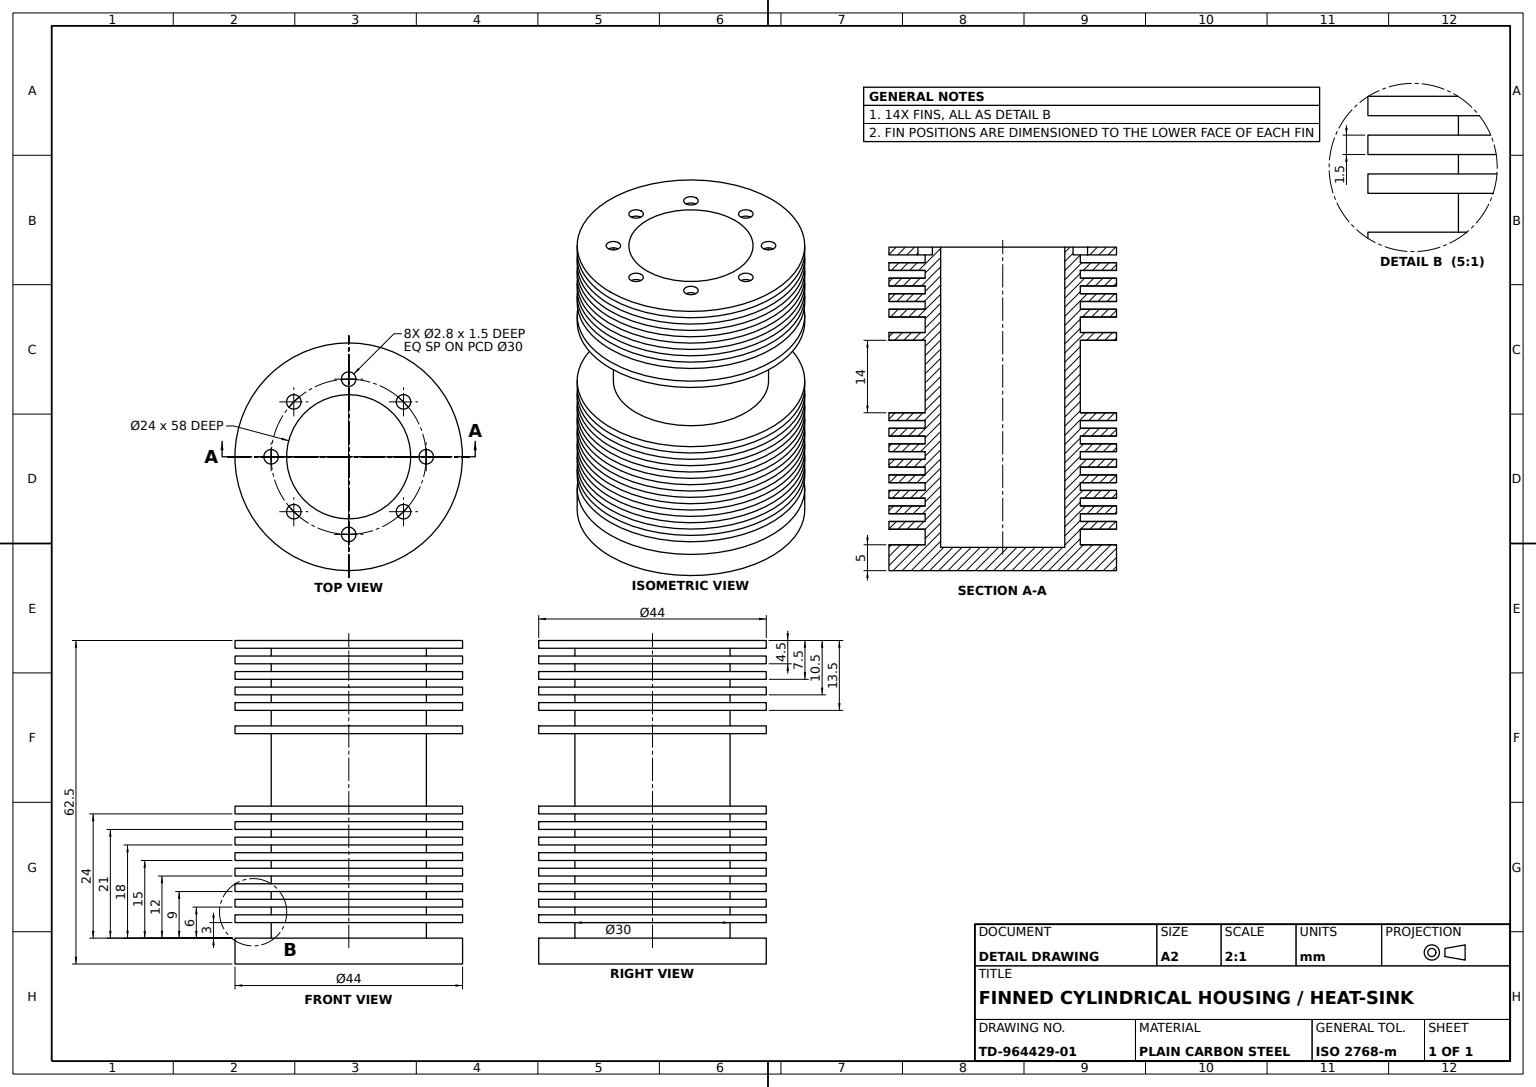
solid
v1 (0,61,13.6)
v2 (0,62.5,13.6)
e1 v1 v2 LINE
v3 (0,62.5,16.4)
e2 v2 v3 CIRCLE(AX(P(0,62.5,15),D(0,1,0),D(0,0,1)),1.4)
v4 (0,61,16.4)
e3 v4 v3 LINE
v5 (-1.398475,61,14.934667)
e4 v5 v4 CIRCLE(AX(P(0,61,15),D(0,1,0),D(0,0,1)),1.4)
e5 v1 v5 CIRCLE(AX(P(0,61,15),D(0,1,0),D(0,0,1)),1.4)
face CYL(AX(P(0,61,15),D(0,1,0),D(0,0,1)),1.4) rev [e1 e2 -e3 -e4 -e5]
v6 (0,15.5,22)
v7 (0,14,22)
e6 v6 v7 LINE
v8 (0,15.5,-22)
e7 v8 v6 CIRCLE(AX(P(0,15.5,0),D(0,1,0),D(0,0,1)),22)
v9 (0,14,-22)
e8 v8 v9 LINE
e9 v9 v7 CIRCLE(AX(P(0,14,0),D(0,1,0),D(0,0,1)),22)
face CYL(AX(P(0,15.5,0),D(0,-1,0),D(0,0,-1)),22) [-e6 -e7 e8 e9]
v10 (0,52,-22)
v11 (0,52,22)
e10 v10 v11 CIRCLE(AX(P(0,52,0),D(0,1,0),D(0,0,1)),22)
v12 (0,53.5,22)
e11 v12 v11 LINE
v13 (0,53.5,-22)
e12 v13 v12 CIRCLE(AX(P(0,53.5,0),D(0,1,0),D(0,0,1)),22)
e13 v13 v10 LINE
face CYL(AX(P(0,53.5,0),D(0,-1,0),D(0,0,-1)),22) [e10 -e11 -e12 e13]
v14 (0,4.5,-12)
v15 (0,4.5,12)
e14 v14 v15 CIRCLE(AX(P(0,4.5,0),D(0,1,0),D(0,0,1)),12)
e15 v15 v14 CIRCLE(AX(P(0,4.5,0),D(0,1,0),D(0,0,1)),12)
face PLANE(AX(P(0,4.5,0),D(0,1,0),D(0,0,1))) [e14 e15]
v16 (0,21.5,15)
v17 (0,21.5,-15)
e16 v16 v17 CIRCLE(AX(P(0,21.5,0),D(0,1,0),D(0,0,1)),15)
v18 (0,23,-15)
e17 v17 v18 LINE
v19 (0,23,15)
e18 v19 v18 CIRCLE(AX(P(0,23,0),D(0,1,0),D(0,0,1)),15)
e19 v16 v19 LINE
face CYL(AX(P(0,4.5,0),D(0,1,0),D(0,0,1)),15) [e16 e17 -e18 -e19]
v20 (-14.934667,61,-1.398475)
v21 (-14.934667,61,1.398475)
e20 v20 v21 CIRCLE(AX(P(0,61,0),D(0,1,0),D(0,0,1)),15)
e21 v21 v20 CIRCLE(AX(P(-15,61,0),D(0,1,0),D(0,0,1)),1.4)
face PLANE(AX(P(-15,61,0),D(0,1,0),D(0,0,1))) [e20 e21]
v22 (10.606602,61,-9.206602)
v23 (11.549275,61,-9.571533)
e22 v22 v23 CIRCLE(AX(P(10.606602,61,-10.606602),D(0,1,0),D(0,0,1)),1.4)
v24 (9.571533,61,-11.549275)
e23 v23 v24 CIRCLE(AX(P(0,61,0),D(0,1,0),D(0,0,1)),15)
e24 v24 v22 CIRCLE(AX(P(10.606602,61,-10.606602),D(0,1,0),D(0,0,1)),1.4)
face PLANE(AX(P(10.606602,61,-10.606602),D(0,1,0),D(0,0,1))) [e22 e23 e24]
v25 (-10.606602,61,9.206602)
v26 (-11.549275,61,9.571533)
e25 v25 v26 CIRCLE(AX(P(-10.606602,61,10.606602),D(0,1,0),D(0,0,1)),1.4)
v27 (-10.606602,62.5,9.206602)
e26 v25 v27 LINE
v28 (-10.606602,62.5,12.006602)
e27 v27 v28 CIRCLE(AX(P(-10.606602,62.5,10.606602),D(0,1,0),D(0,0,1)),1.4)
v29 (-10.606602,61,12.006602)
e28 v29 v28 LINE
e29 v26 v29 CIRCLE(AX(P(-10.606602,61,10.606602),D(0,1,0),D(0,0,1)),1.4)
face CYL(AX(P(-10.606602,61,10.606602),D(0,1,0),D(0,0,1)),1.4) rev [-e25 e26 e27 -e28 -e29]
v30 (-9.571533,61,-11.549275)
v31 (-11.549275,61,-9.571533)
e30 v30 v31 CIRCLE(AX(P(0,61,0),D(0,1,0),D(0,0,1)),15)
v32 (-10.606602,61,-9.206602)
e31 v31 v32 CIRCLE(AX(P(-10.606602,61,-10.606602),D(0,1,0),D(0,0,1)),1.4)
e32 v32 v30 CIRCLE(AX(P(-10.606602,61,-10.606602),D(0,1,0),D(0,0,1)),1.4)
face PLANE(AX(P(-10.606602,61,-10.606602),D(0,1,0),D(0,0,1))) [e30 e31 e32]
v33 (0,50.5,-15)
v34 (0,52,-15)
e33 v33 v34 LINE
v35 (0,52,15)
e34 v35 v34 CIRCLE(AX(P(0,52,0),D(0,1,0),D(0,0,1)),15)
v36 (0,50.5,15)
e35 v36 v35 LINE
e36 v36 v33 CIRCLE(AX(P(0,50.5,0),D(0,1,0),D(0,0,1)),15)
face CYL(AX(P(0,4.5,0),D(0,1,0),D(0,0,1)),15) [e33 -e34 -e35 e36]
e37 v12 v13 CIRCLE(AX(P(0,53.5,0),D(0,1,0),D(0,0,1)),22)
e38 v11 v10 CIRCLE(AX(P(0,52,0),D(0,1,0),D(0,0,1)),22)
face CYL(AX(P(0,53.5,0),D(0,-1,0),D(0,0,-1)),22) [-e13 -e37 e11 e38]
v37 (-15,61,-1.4)
e39 v20 v37 CIRCLE(AX(P(-15,61,0),D(0,1,0),D(0,0,1)),1.4)
v38 (-15,61,1.4)
e40 v37 v38 CIRCLE(AX(P(-15,61,0),D(0,1,0),D(0,0,1)),1.4)
e41 v38 v21 CIRCLE(AX(P(-15,61,0),D(0,1,0),D(0,0,1)),1.4)
e42 v21 v26 CIRCLE(AX(P(0,61,0),D(0,1,0),D(0,0,1)),15)
v39 (-9.571533,61,11.549275)
e43 v29 v39 CIRCLE(AX(P(-10.606602,61,10.606602),D(0,1,0),D(0,0,1)),1.4)
e44 v39 v5 CIRCLE(AX(P(0,61,0),D(0,1,0),D(0,0,1)),15)
v40 (1.398475,61,14.934667)
e45 v4 v40 CIRCLE(AX(P(0,61,15),D(0,1,0),D(0,0,1)),1.4)
v41 (9.571533,61,11.549275)
e46 v40 v41 CIRCLE(AX(P(0,61,0),D(0,1,0),D(0,0,1)),15)
v42 (10.606602,61,12.006602)
e47 v41 v42 CIRCLE(AX(P(10.606602,61,10.606602),D(0,1,0),D(0,0,1)),1.4)
v43 (11.549275,61,9.571533)
e48 v42 v43 CIRCLE(AX(P(10.606602,61,10.606602),D(0,1,0),D(0,0,1)),1.4)
v44 (14.934667,61,1.398475)
e49 v43 v44 CIRCLE(AX(P(0,61,0),D(0,1,0),D(0,0,1)),15)
v45 (15,61,1.4)
e50 v44 v45 CIRCLE(AX(P(15,61,0),D(0,1,0),D(0,0,1)),1.4)
v46 (15,61,-1.4)
e51 v45 v46 CIRCLE(AX(P(15,61,0),D(0,1,0),D(0,0,1)),1.4)
v47 (14.934667,61,-1.398475)
e52 v46 v47 CIRCLE(AX(P(15,61,0),D(0,1,0),D(0,0,1)),1.4)
e53 v47 v23 CIRCLE(AX(P(0,61,0),D(0,1,0),D(0,0,1)),15)
v48 (10.606602,61,-12.006602)
e54 v23 v48 CIRCLE(AX(P(10.606602,61,-10.606602),D(0,1,0),D(0,0,1)),1.4)
e55 v48 v24 CIRCLE(AX(P(10.606602,61,-10.606602),D(0,1,0),D(0,0,1)),1.4)
v49 (1.398475,61,-14.934667)
e56 v24 v49 CIRCLE(AX(P(0,61,0),D(0,1,0),D(0,0,1)),15)
v50 (0,61,-16.4)
e57 v49 v50 CIRCLE(AX(P(0,61,-15),D(0,1,0),D(0,0,1)),1.4)
v51 (-1.398475,61,-14.934667)
e58 v50 v51 CIRCLE(AX(P(0,61,-15),D(0,1,0),D(0,0,1)),1.4)
e59 v51 v30 CIRCLE(AX(P(0,61,0),D(0,1,0),D(0,0,1)),15)
v52 (-10.606602,61,-12.006602)
e60 v30 v52 CIRCLE(AX(P(-10.606602,61,-10.606602),D(0,1,0),D(0,0,1)),1.4)
e61 v52 v31 CIRCLE(AX(P(-10.606602,61,-10.606602),D(0,1,0),D(0,0,1)),1.4)
e62 v31 v20 CIRCLE(AX(P(0,61,0),D(0,1,0),D(0,0,1)),15)
v53 (0,61,22)
v54 (0,61,-22)
e63 v53 v54 CIRCLE(AX(P(0,61,0),D(0,1,0),D(0,0,1)),22)
e64 v54 v53 CIRCLE(AX(P(0,61,0),D(0,1,0),D(0,0,1)),22)
face PLANE(AX(P(0,61,0),D(0,1,0),D(0,0,1))) rev [e39 e40 e41 e42 e29 e43 e44 e4 e45 e46 e47 e48 e49 e50 e51 e52 e53 e54 e55 e56 e57 e58 e59 e60 e61 e62] [-e63 -e64]
v55 (0,49,15)
v56 (0,49,-15)
e65 v55 v56 CIRCLE(AX(P(0,49,0),D(0,1,0),D(0,0,1)),15)
v57 (0,46,15)
e66 v57 v55 LINE
v58 (0,46,-15)
e67 v57 v58 CIRCLE(AX(P(0,46,0),D(0,1,0),D(0,0,1)),15)
e68 v58 v56 LINE
face CYL(AX(P(0,4.5,0),D(0,1,0),D(0,0,1)),15) [-e65 -e66 e67 e68]
v59 (0,21.5,22)
v60 (0,20,22)
e69 v59 v60 LINE
v61 (0,21.5,-22)
e70 v61 v59 CIRCLE(AX(P(0,21.5,0),D(0,1,0),D(0,0,1)),22)
v62 (0,20,-22)
e71 v61 v62 LINE
e72 v62 v60 CIRCLE(AX(P(0,20,0),D(0,1,0),D(0,0,1)),22)
face CYL(AX(P(0,21.5,0),D(0,-1,0),D(0,0,-1)),22) [-e69 -e70 e71 e72]
v63 (15,62.5,1.4)
e73 v45 v63 LINE
v64 (15,62.5,-1.4)
e74 v63 v64 CIRCLE(AX(P(15,62.5,0),D(0,1,0),D(0,0,1)),1.4)
e75 v46 v64 LINE
face CYL(AX(P(15,61,0),D(0,1,0),D(0,0,1)),1.4) rev [e73 e74 -e75 -e51]
v65 (0,0,22)
v66 (0,0,-22)
e76 v65 v66 CIRCLE(AX(P(0,0,0),D(0,1,0),D(0,0,1)),22)
e77 v66 v65 CIRCLE(AX(P(0,0,0),D(0,1,0),D(0,0,1)),22)
face PLANE(AX(P(0,0,0),D(0,1,0),D(0,0,1))) rev [-e76 -e77]
v67 (0,30.5,-15)
v68 (0,44.5,-15)
e78 v67 v68 LINE
v69 (0,30.5,15)
e79 v67 v69 CIRCLE(AX(P(0,30.5,0),D(0,1,0),D(0,0,1)),15)
v70 (0,44.5,15)
e80 v69 v70 LINE
e81 v68 v70 CIRCLE(AX(P(0,44.5,0),D(0,1,0),D(0,0,1)),15)
face CYL(AX(P(0,4.5,0),D(0,1,0),D(0,0,1)),15) [-e78 e79 e80 -e81]
v71 (0,17,22)
v72 (0,17,-22)
e82 v71 v72 CIRCLE(AX(P(0,17,0),D(0,1,0),D(0,0,1)),22)
v73 (0,18.5,-22)
e83 v73 v72 LINE
v74 (0,18.5,22)
e84 v74 v73 CIRCLE(AX(P(0,18.5,0),D(0,1,0),D(0,0,1)),22)
e85 v74 v71 LINE
face CYL(AX(P(0,18.5,0),D(0,-1,0),D(0,0,-1)),22) [e82 -e83 -e84 e85]
v75 (0,29,-22)
v76 (0,29,22)
e86 v75 v76 CIRCLE(AX(P(0,29,0),D(0,1,0),D(0,0,1)),22)
v77 (0,30.5,22)
e87 v77 v76 LINE
v78 (0,30.5,-22)
e88 v78 v77 CIRCLE(AX(P(0,30.5,0),D(0,1,0),D(0,0,1)),22)
e89 v78 v75 LINE
face CYL(AX(P(0,30.5,0),D(0,-1,0),D(0,0,-1)),22) [e86 -e87 -e88 e89]
e90 v59 v61 CIRCLE(AX(P(0,21.5,0),D(0,1,0),D(0,0,1)),22)
e91 v17 v16 CIRCLE(AX(P(0,21.5,0),D(0,1,0),D(0,0,1)),15)
face PLANE(AX(P(0,21.5,0),D(0,1,0),D(0,0,1))) [e70 e90] [-e91 -e16]
e92 v40 v1 CIRCLE(AX(P(0,61,15),D(0,1,0),D(0,0,1)),1.4)
e93 v3 v2 CIRCLE(AX(P(0,62.5,15),D(0,1,0),D(0,0,1)),1.4)
face CYL(AX(P(0,61,15),D(0,1,0),D(0,0,1)),1.4) rev [-e1 -e92 -e45 e3 e93]
e94 v60 v62 CIRCLE(AX(P(0,20,0),D(0,1,0),D(0,0,1)),22)
face CYL(AX(P(0,21.5,0),D(0,-1,0),D(0,0,-1)),22) [e94 -e71 -e90 e69]
v79 (0,11,-15)
v80 (0,11,15)
e95 v79 v80 CIRCLE(AX(P(0,11,0),D(0,1,0),D(0,0,1)),15)
v81 (0,9.5,-15)
e96 v81 v79 LINE
v82 (0,9.5,15)
e97 v81 v82 CIRCLE(AX(P(0,9.5,0),D(0,1,0),D(0,0,1)),15)
e98 v82 v80 LINE
face CYL(AX(P(0,4.5,0),D(0,1,0),D(0,0,1)),15) [-e95 -e96 e97 e98]
v83 (0,20,-15)
v84 (0,20,15)
e99 v83 v84 CIRCLE(AX(P(0,20,0),D(0,1,0),D(0,0,1)),15)
e100 v84 v83 CIRCLE(AX(P(0,20,0),D(0,1,0),D(0,0,1)),15)
face PLANE(AX(P(0,20,0),D(0,1,0),D(0,0,1))) rev [-e94 -e72] [e99 e100]
e101 v39 v25 CIRCLE(AX(P(-10.606602,61,10.606602),D(0,1,0),D(0,0,1)),1.4)
e102 v26 v39 CIRCLE(AX(P(0,61,0),D(0,1,0),D(0,0,1)),15)
face PLANE(AX(P(-10.606602,61,10.606602),D(0,1,0),D(0,0,1))) [e101 e25 e102]
e103 v34 v35 CIRCLE(AX(P(0,52,0),D(0,1,0),D(0,0,1)),15)
e104 v33 v36 CIRCLE(AX(P(0,50.5,0),D(0,1,0),D(0,0,1)),15)
face CYL(AX(P(0,4.5,0),D(0,1,0),D(0,0,1)),15) [e35 -e103 -e33 e104]
v85 (0,59.5,15)
v86 (0,59.5,-15)
e105 v85 v86 CIRCLE(AX(P(0,59.5,0),D(0,1,0),D(0,0,1)),15)
e106 v86 v85 CIRCLE(AX(P(0,59.5,0),D(0,1,0),D(0,0,1)),15)
v87 (0,59.5,22)
v88 (0,59.5,-22)
e107 v87 v88 CIRCLE(AX(P(0,59.5,0),D(0,1,0),D(0,0,1)),22)
e108 v88 v87 CIRCLE(AX(P(0,59.5,0),D(0,1,0),D(0,0,1)),22)
face PLANE(AX(P(0,59.5,0),D(0,1,0),D(0,0,1))) [-e105 -e106] [e107 e108]
e109 v77 v78 CIRCLE(AX(P(0,30.5,0),D(0,1,0),D(0,0,1)),22)
e110 v69 v67 CIRCLE(AX(P(0,30.5,0),D(0,1,0),D(0,0,1)),15)
face PLANE(AX(P(0,30.5,0),D(0,1,0),D(0,0,1))) [e109 e88] [-e79 -e110]
v89 (-15,62.5,1.4)
e111 v38 v89 LINE
v90 (-15,62.5,-1.4)
e112 v89 v90 CIRCLE(AX(P(-15,62.5,0),D(0,1,0),D(0,0,1)),1.4)
e113 v37 v90 LINE
face CYL(AX(P(-15,61,0),D(0,1,0),D(0,0,1)),1.4) rev [-e39 -e21 -e41 e111 e112 -e113]
v91 (0,56.5,15)
v92 (0,58,15)
e114 v91 v92 LINE
v93 (0,58,-15)
e115 v93 v92 CIRCLE(AX(P(0,58,0),D(0,1,0),D(0,0,1)),15)
v94 (0,56.5,-15)
e116 v94 v93 LINE
e117 v94 v91 CIRCLE(AX(P(0,56.5,0),D(0,1,0),D(0,0,1)),15)
face CYL(AX(P(0,4.5,0),D(0,1,0),D(0,0,1)),15) [e114 -e115 -e116 e117]
v95 (0,62.5,-16.4)
e118 v50 v95 LINE
v96 (0,62.5,-13.6)
e119 v95 v96 CIRCLE(AX(P(0,62.5,-15),D(0,1,0),D(0,0,1)),1.4)
v97 (0,61,-13.6)
e120 v97 v96 LINE
e121 v51 v97 CIRCLE(AX(P(0,61,-15),D(0,1,0),D(0,0,1)),1.4)
face CYL(AX(P(0,61,-15),D(0,1,0),D(0,0,1)),1.4) rev [e118 e119 -e120 -e121 -e58]
e122 v82 v81 CIRCLE(AX(P(0,9.5,0),D(0,1,0),D(0,0,1)),15)
v98 (0,9.5,22)
v99 (0,9.5,-22)
e123 v98 v99 CIRCLE(AX(P(0,9.5,0),D(0,1,0),D(0,0,1)),22)
e124 v99 v98 CIRCLE(AX(P(0,9.5,0),D(0,1,0),D(0,0,1)),22)
face PLANE(AX(P(0,9.5,0),D(0,1,0),D(0,0,1))) [-e97 -e122] [e123 e124]
e125 v73 v74 CIRCLE(AX(P(0,18.5,0),D(0,1,0),D(0,0,1)),22)
v100 (0,18.5,15)
v101 (0,18.5,-15)
e126 v100 v101 CIRCLE(AX(P(0,18.5,0),D(0,1,0),D(0,0,1)),15)
e127 v101 v100 CIRCLE(AX(P(0,18.5,0),D(0,1,0),D(0,0,1)),15)
face PLANE(AX(P(0,18.5,0),D(0,1,0),D(0,0,1))) [e84 e125] [-e126 -e127]
e128 v6 v8 CIRCLE(AX(P(0,15.5,0),D(0,1,0),D(0,0,1)),22)
e129 v7 v9 CIRCLE(AX(P(0,14,0),D(0,1,0),D(0,0,1)),22)
face CYL(AX(P(0,15.5,0),D(0,-1,0),D(0,0,-1)),22) [-e8 -e128 e6 e129]
e130 v72 v71 CIRCLE(AX(P(0,17,0),D(0,1,0),D(0,0,1)),22)
face CYL(AX(P(0,18.5,0),D(0,-1,0),D(0,0,-1)),22) [e83 e130 -e85 -e125]
v102 (0,61,-15)
e131 v86 v102 LINE
v103 (0,61,15)
e132 v85 v103 LINE
e133 v5 v103 CIRCLE(AX(P(0,61,0),D(0,1,0),D(0,0,1)),15)
e134 v102 v51 CIRCLE(AX(P(0,61,0),D(0,1,0),D(0,0,1)),15)
face CYL(AX(P(0,4.5,0),D(0,1,0),D(0,0,1)),15) [-e131 e106 e132 -e133 -e44 -e102 -e42 -e20 -e62 -e30 -e59 -e134]
v104 (0,12.5,-15)
v105 (0,14,-15)
e135 v104 v105 LINE
v106 (0,12.5,15)
e136 v104 v106 CIRCLE(AX(P(0,12.5,0),D(0,1,0),D(0,0,1)),15)
v107 (0,14,15)
e137 v106 v107 LINE
e138 v105 v107 CIRCLE(AX(P(0,14,0),D(0,1,0),D(0,0,1)),15)
face CYL(AX(P(0,4.5,0),D(0,1,0),D(0,0,1)),15) [-e135 e136 e137 -e138]
v108 (0,5,-22)
e139 v108 v66 LINE
v109 (0,5,22)
e140 v109 v65 LINE
e141 v108 v109 CIRCLE(AX(P(0,5,0),D(0,1,0),D(0,0,1)),22)
face CYL(AX(P(0,5,0),D(0,-1,0),D(0,0,-1)),22) [e139 e77 -e140 -e141]
v110 (0,46,-22)
v111 (0,44.5,-22)
e142 v110 v111 LINE
v112 (0,46,22)
e143 v112 v110 CIRCLE(AX(P(0,46,0),D(0,1,0),D(0,0,1)),22)
v113 (0,44.5,22)
e144 v112 v113 LINE
e145 v113 v111 CIRCLE(AX(P(0,44.5,0),D(0,1,0),D(0,0,1)),22)
face CYL(AX(P(0,46,0),D(0,-1,0),D(0,0,-1)),22) [-e142 -e143 e144 e145]
v114 (0,15.5,-15)
v115 (0,15.5,15)
e146 v114 v115 CIRCLE(AX(P(0,15.5,0),D(0,1,0),D(0,0,1)),15)
e147 v115 v114 CIRCLE(AX(P(0,15.5,0),D(0,1,0),D(0,0,1)),15)
face PLANE(AX(P(0,15.5,0),D(0,1,0),D(0,0,1))) [e7 e128] [-e146 -e147]
e148 v70 v68 CIRCLE(AX(P(0,44.5,0),D(0,1,0),D(0,0,1)),15)
e149 v111 v113 CIRCLE(AX(P(0,44.5,0),D(0,1,0),D(0,0,1)),22)
face PLANE(AX(P(0,44.5,0),D(0,1,0),D(0,0,1))) rev [e148 e81] [-e149 -e145]
v116 (0,24.5,15)
v117 (0,26,15)
e150 v116 v117 LINE
v118 (0,24.5,-15)
e151 v116 v118 CIRCLE(AX(P(0,24.5,0),D(0,1,0),D(0,0,1)),15)
v119 (0,26,-15)
e152 v118 v119 LINE
e153 v117 v119 CIRCLE(AX(P(0,26,0),D(0,1,0),D(0,0,1)),15)
face CYL(AX(P(0,4.5,0),D(0,1,0),D(0,0,1)),15) [-e150 e151 e152 -e153]
e154 v119 v117 CIRCLE(AX(P(0,26,0),D(0,1,0),D(0,0,1)),15)
e155 v118 v116 CIRCLE(AX(P(0,24.5,0),D(0,1,0),D(0,0,1)),15)
face CYL(AX(P(0,4.5,0),D(0,1,0),D(0,0,1)),15) [-e154 -e152 e155 e150]
e156 v107 v105 CIRCLE(AX(P(0,14,0),D(0,1,0),D(0,0,1)),15)
face PLANE(AX(P(0,14,0),D(0,1,0),D(0,0,1))) rev [e138 e156] [-e129 -e9]
v120 (0,5,-15)
v121 (0,5,15)
e157 v120 v121 CIRCLE(AX(P(0,5,0),D(0,1,0),D(0,0,1)),15)
v122 (0,8,15)
e158 v121 v122 LINE
v123 (0,8,-15)
e159 v123 v122 CIRCLE(AX(P(0,8,0),D(0,1,0),D(0,0,1)),15)
e160 v120 v123 LINE
face CYL(AX(P(0,4.5,0),D(0,1,0),D(0,0,1)),15) [e157 e158 -e159 -e160]
v124 (0,62.5,-22)
e161 v124 v54 LINE
v125 (0,62.5,22)
e162 v125 v124 CIRCLE(AX(P(0,62.5,0),D(0,1,0),D(0,0,1)),22)
e163 v125 v53 LINE
face CYL(AX(P(0,62.5,0),D(0,-1,0),D(0,0,-1)),22) [-e161 -e162 e163 e63]
e164 v92 v93 CIRCLE(AX(P(0,58,0),D(0,1,0),D(0,0,1)),15)
e165 v91 v94 CIRCLE(AX(P(0,56.5,0),D(0,1,0),D(0,0,1)),15)
face CYL(AX(P(0,4.5,0),D(0,1,0),D(0,0,1)),15) [-e164 -e114 e165 e116]
v126 (0,53.5,-15)
v127 (0,53.5,15)
e166 v126 v127 CIRCLE(AX(P(0,53.5,0),D(0,1,0),D(0,0,1)),15)
e167 v127 v126 CIRCLE(AX(P(0,53.5,0),D(0,1,0),D(0,0,1)),15)
face PLANE(AX(P(0,53.5,0),D(0,1,0),D(0,0,1))) [-e166 -e167] [e37 e12]
e168 v18 v19 CIRCLE(AX(P(0,23,0),D(0,1,0),D(0,0,1)),15)
face CYL(AX(P(0,4.5,0),D(0,1,0),D(0,0,1)),15) [-e168 -e17 e91 e19]
v128 (10.606602,61,9.206602)
e169 v128 v41 CIRCLE(AX(P(10.606602,61,10.606602),D(0,1,0),D(0,0,1)),1.4)
v129 (10.606602,62.5,9.206602)
e170 v128 v129 LINE
v130 (10.606602,62.5,12.006602)
e171 v129 v130 CIRCLE(AX(P(10.606602,62.5,10.606602),D(0,1,0),D(0,0,1)),1.4)
e172 v42 v130 LINE
face CYL(AX(P(10.606602,61,10.606602),D(0,1,0),D(0,0,1)),1.4) rev [-e47 -e169 e170 e171 -e172]
e173 v106 v104 CIRCLE(AX(P(0,12.5,0),D(0,1,0),D(0,0,1)),15)
v131 (0,12.5,-22)
v132 (0,12.5,22)
e174 v131 v132 CIRCLE(AX(P(0,12.5,0),D(0,1,0),D(0,0,1)),22)
e175 v132 v131 CIRCLE(AX(P(0,12.5,0),D(0,1,0),D(0,0,1)),22)
face PLANE(AX(P(0,12.5,0),D(0,1,0),D(0,0,1))) [-e136 -e173] [e174 e175]
v133 (0,55,-15)
v134 (0,55,15)
e176 v133 v134 CIRCLE(AX(P(0,55,0),D(0,1,0),D(0,0,1)),15)
e177 v126 v133 LINE
e178 v127 v134 LINE
face CYL(AX(P(0,4.5,0),D(0,1,0),D(0,0,1)),15) [-e176 -e177 e166 e178]
e179 v130 v129 CIRCLE(AX(P(10.606602,62.5,10.606602),D(0,1,0),D(0,0,1)),1.4)
e180 v43 v128 CIRCLE(AX(P(10.606602,61,10.606602),D(0,1,0),D(0,0,1)),1.4)
face CYL(AX(P(10.606602,61,10.606602),D(0,1,0),D(0,0,1)),1.4) rev [e179 -e170 -e180 -e48 e172]
e181 v58 v57 CIRCLE(AX(P(0,46,0),D(0,1,0),D(0,0,1)),15)
e182 v110 v112 CIRCLE(AX(P(0,46,0),D(0,1,0),D(0,0,1)),22)
face PLANE(AX(P(0,46,0),D(0,1,0),D(0,0,1))) [-e181 -e67] [e143 e182]
v135 (0,27.5,-22)
v136 (0,26,-22)
e183 v135 v136 LINE
v137 (0,26,22)
e184 v136 v137 CIRCLE(AX(P(0,26,0),D(0,1,0),D(0,0,1)),22)
v138 (0,27.5,22)
e185 v138 v137 LINE
e186 v135 v138 CIRCLE(AX(P(0,27.5,0),D(0,1,0),D(0,0,1)),22)
face CYL(AX(P(0,27.5,0),D(0,-1,0),D(0,0,-1)),22) [e183 e184 -e185 -e186]
v139 (0,24.5,22)
v140 (0,24.5,-22)
e187 v139 v140 CIRCLE(AX(P(0,24.5,0),D(0,1,0),D(0,0,1)),22)
v141 (0,23,22)
e188 v139 v141 LINE
v142 (0,23,-22)
e189 v141 v142 CIRCLE(AX(P(0,23,0),D(0,1,0),D(0,0,1)),22)
e190 v140 v142 LINE
face CYL(AX(P(0,24.5,0),D(0,-1,0),D(0,0,-1)),22) [-e187 e188 e189 -e190]
e191 v76 v75 CIRCLE(AX(P(0,29,0),D(0,1,0),D(0,0,1)),22)
face CYL(AX(P(0,30.5,0),D(0,-1,0),D(0,0,-1)),22) [e191 -e89 -e109 e87]
e192 v90 v89 CIRCLE(AX(P(-15,62.5,0),D(0,1,0),D(0,0,1)),1.4)
face CYL(AX(P(-15,61,0),D(0,1,0),D(0,0,1)),1.4) rev [-e40 e113 e192 -e111]
e193 v41 v43 CIRCLE(AX(P(0,61,0),D(0,1,0),D(0,0,1)),15)
face PLANE(AX(P(10.606602,61,10.606602),D(0,1,0),D(0,0,1))) [e180 e169 e193]
face CYL(AX(P(0,4.5,0),D(0,1,0),D(0,0,1)),15) [e110 e78 -e148 -e80]
v143 (0,8,22)
e194 v98 v143 LINE
v144 (0,8,-22)
e195 v99 v144 LINE
e196 v144 v143 CIRCLE(AX(P(0,8,0),D(0,1,0),D(0,0,1)),22)
face CYL(AX(P(0,9.5,0),D(0,-1,0),D(0,0,-1)),22) [-e194 -e124 e195 e196]
e197 v138 v135 CIRCLE(AX(P(0,27.5,0),D(0,1,0),D(0,0,1)),22)
e198 v137 v136 CIRCLE(AX(P(0,26,0),D(0,1,0),D(0,0,1)),22)
face CYL(AX(P(0,27.5,0),D(0,-1,0),D(0,0,-1)),22) [-e183 -e197 e185 e198]
e199 v47 v44 CIRCLE(AX(P(15,61,0),D(0,1,0),D(0,0,1)),1.4)
e200 v64 v63 CIRCLE(AX(P(15,62.5,0),D(0,1,0),D(0,0,1)),1.4)
face CYL(AX(P(15,61,0),D(0,1,0),D(0,0,1)),1.4) rev [-e73 -e50 -e199 -e52 e75 e200]
v145 (0,17,-15)
v146 (0,17,15)
e201 v145 v146 CIRCLE(AX(P(0,17,0),D(0,1,0),D(0,0,1)),15)
e202 v146 v145 CIRCLE(AX(P(0,17,0),D(0,1,0),D(0,0,1)),15)
face PLANE(AX(P(0,17,0),D(0,1,0),D(0,0,1))) rev [e201 e202] [-e82 -e130]
v147 (0,58,22)
v148 (0,58,-22)
e203 v147 v148 CIRCLE(AX(P(0,58,0),D(0,1,0),D(0,0,1)),22)
e204 v148 v147 CIRCLE(AX(P(0,58,0),D(0,1,0),D(0,0,1)),22)
face PLANE(AX(P(0,58,0),D(0,1,0),D(0,0,1))) rev [-e203 -e204] [e115 e164]
face CYL(AX(P(0,4.5,0),D(0,1,0),D(0,0,1)),15) [-e156 -e137 e173 e135]
v149 (0,11,-22)
e205 v131 v149 LINE
v150 (0,11,22)
e206 v132 v150 LINE
e207 v150 v149 CIRCLE(AX(P(0,11,0),D(0,1,0),D(0,0,1)),22)
face CYL(AX(P(0,12.5,0),D(0,-1,0),D(0,0,-1)),22) [-e205 -e175 e206 e207]
v151 (0,27.5,-15)
v152 (0,29,-15)
e208 v151 v152 LINE
v153 (0,29,15)
e209 v153 v152 CIRCLE(AX(P(0,29,0),D(0,1,0),D(0,0,1)),15)
v154 (0,27.5,15)
e210 v154 v153 LINE
e211 v154 v151 CIRCLE(AX(P(0,27.5,0),D(0,1,0),D(0,0,1)),15)
face CYL(AX(P(0,4.5,0),D(0,1,0),D(0,0,1)),15) [e208 -e209 -e210 e211]
e212 v143 v144 CIRCLE(AX(P(0,8,0),D(0,1,0),D(0,0,1)),22)
face CYL(AX(P(0,9.5,0),D(0,-1,0),D(0,0,-1)),22) [e194 e212 -e195 -e123]
e213 v100 v84 LINE
e214 v101 v83 LINE
face CYL(AX(P(0,4.5,0),D(0,1,0),D(0,0,1)),15) [-e100 -e213 e126 e214]
e215 v28 v27 CIRCLE(AX(P(-10.606602,62.5,10.606602),D(0,1,0),D(0,0,1)),1.4)
face CYL(AX(P(-10.606602,61,10.606602),D(0,1,0),D(0,0,1)),1.4) rev [-e101 -e43 e28 e215 -e26]
v155 (0,56.5,-22)
v156 (0,56.5,22)
e216 v155 v156 CIRCLE(AX(P(0,56.5,0),D(0,1,0),D(0,0,1)),22)
v157 (0,55,-22)
e217 v155 v157 LINE
v158 (0,55,22)
e218 v157 v158 CIRCLE(AX(P(0,55,0),D(0,1,0),D(0,0,1)),22)
e219 v156 v158 LINE
face CYL(AX(P(0,56.5,0),D(0,-1,0),D(0,0,-1)),22) [-e216 e217 e218 -e219]
e220 v80 v79 CIRCLE(AX(P(0,11,0),D(0,1,0),D(0,0,1)),15)
face CYL(AX(P(0,4.5,0),D(0,1,0),D(0,0,1)),15) [-e220 -e98 e122 e96]
e221 v124 v125 CIRCLE(AX(P(0,62.5,0),D(0,1,0),D(0,0,1)),22)
face CYL(AX(P(0,62.5,0),D(0,-1,0),D(0,0,-1)),22) [-e221 e161 e64 -e163]
e222 v87 v147 LINE
e223 v88 v148 LINE
face CYL(AX(P(0,59.5,0),D(0,-1,0),D(0,0,-1)),22) [-e222 -e108 e223 e204]
e224 v109 v108 CIRCLE(AX(P(0,5,0),D(0,1,0),D(0,0,1)),22)
face CYL(AX(P(0,5,0),D(0,-1,0),D(0,0,-1)),22) [-e224 e140 e76 -e139]
e225 v121 v120 CIRCLE(AX(P(0,5,0),D(0,1,0),D(0,0,1)),15)
face PLANE(AX(P(0,5,0),D(0,1,0),D(0,0,1))) [-e157 -e225] [e224 e141]
face CYL(AX(P(0,4.5,0),D(0,1,0),D(0,0,1)),15) [e127 e213 -e99 -e214]
face CYL(AX(P(0,59.5,0),D(0,-1,0),D(0,0,-1)),22) [-e107 e222 e203 -e223]
e226 v151 v154 CIRCLE(AX(P(0,27.5,0),D(0,1,0),D(0,0,1)),15)
face PLANE(AX(P(0,27.5,0),D(0,1,0),D(0,0,1))) [e186 e197] [-e226 -e211]
e227 v122 v123 CIRCLE(AX(P(0,8,0),D(0,1,0),D(0,0,1)),15)
face CYL(AX(P(0,4.5,0),D(0,1,0),D(0,0,1)),15) [-e227 -e158 e225 e160]
e228 v152 v153 CIRCLE(AX(P(0,29,0),D(0,1,0),D(0,0,1)),15)
face CYL(AX(P(0,4.5,0),D(0,1,0),D(0,0,1)),15) [e226 e210 -e228 -e208]
face PLANE(AX(P(0,8,0),D(0,1,0),D(0,0,1))) rev [e227 e159] [-e196 -e212]
v159 (0,50.5,-22)
v160 (0,49,-22)
e229 v159 v160 LINE
v161 (0,49,22)
e230 v160 v161 CIRCLE(AX(P(0,49,0),D(0,1,0),D(0,0,1)),22)
v162 (0,50.5,22)
e231 v162 v161 LINE
e232 v159 v162 CIRCLE(AX(P(0,50.5,0),D(0,1,0),D(0,0,1)),22)
face CYL(AX(P(0,50.5,0),D(0,-1,0),D(0,0,-1)),22) [e229 e230 -e231 -e232]
e233 v149 v150 CIRCLE(AX(P(0,11,0),D(0,1,0),D(0,0,1)),22)
face PLANE(AX(P(0,11,0),D(0,1,0),D(0,0,1))) rev [-e207 -e233] [e220 e95]
v163 (10.606602,62.5,-9.206602)
e234 v22 v163 LINE
v164 (10.606602,62.5,-12.006602)
e235 v163 v164 CIRCLE(AX(P(10.606602,62.5,-10.606602),D(0,1,0),D(0,0,1)),1.4)
e236 v48 v164 LINE
face CYL(AX(P(10.606602,61,-10.606602),D(0,1,0),D(0,0,1)),1.4) rev [-e54 -e22 e234 e235 -e236]
e237 v142 v141 CIRCLE(AX(P(0,23,0),D(0,1,0),D(0,0,1)),22)
e238 v140 v139 CIRCLE(AX(P(0,24.5,0),D(0,1,0),D(0,0,1)),22)
face CYL(AX(P(0,24.5,0),D(0,-1,0),D(0,0,-1)),22) [e237 -e188 -e238 e190]
face PLANE(AX(P(0,24.5,0),D(0,1,0),D(0,0,1))) [-e151 -e155] [e187 e238]
e239 v44 v47 CIRCLE(AX(P(0,61,0),D(0,1,0),D(0,0,1)),15)
face PLANE(AX(P(15,61,0),D(0,1,0),D(0,0,1))) [e239 e199]
e240 v156 v155 CIRCLE(AX(P(0,56.5,0),D(0,1,0),D(0,0,1)),22)
e241 v158 v157 CIRCLE(AX(P(0,55,0),D(0,1,0),D(0,0,1)),22)
face CYL(AX(P(0,56.5,0),D(0,-1,0),D(0,0,-1)),22) [-e240 e219 e241 -e217]
e242 v56 v55 CIRCLE(AX(P(0,49,0),D(0,1,0),D(0,0,1)),15)
face CYL(AX(P(0,4.5,0),D(0,1,0),D(0,0,1)),15) [e181 e66 -e242 -e68]
v165 (-10.606602,62.5,-9.206602)
e243 v32 v165 LINE
v166 (-10.606602,62.5,-12.006602)
e244 v52 v166 LINE
e245 v166 v165 CIRCLE(AX(P(-10.606602,62.5,-10.606602),D(0,1,0),D(0,0,1)),1.4)
face CYL(AX(P(-10.606602,61,-10.606602),D(0,1,0),D(0,0,1)),1.4) rev [-e243 -e31 -e61 e244 e245]
e246 v161 v160 CIRCLE(AX(P(0,49,0),D(0,1,0),D(0,0,1)),22)
e247 v162 v159 CIRCLE(AX(P(0,50.5,0),D(0,1,0),D(0,0,1)),22)
face CYL(AX(P(0,50.5,0),D(0,-1,0),D(0,0,-1)),22) [e231 e246 -e229 -e247]
face PLANE(AX(P(0,26,0),D(0,1,0),D(0,0,1))) rev [e153 e154] [-e184 -e198]
face CYL(AX(P(0,46,0),D(0,-1,0),D(0,0,-1)),22) [e149 -e144 -e182 e142]
face PLANE(AX(P(0,23,0),D(0,1,0),D(0,0,1))) rev [e168 e18] [-e237 -e189]
e248 v97 v49 CIRCLE(AX(P(0,61,-15),D(0,1,0),D(0,0,1)),1.4)
e249 v96 v95 CIRCLE(AX(P(0,62.5,-15),D(0,1,0),D(0,0,1)),1.4)
face CYL(AX(P(0,61,-15),D(0,1,0),D(0,0,1)),1.4) rev [-e57 -e248 e120 e249 -e118]
e250 v165 v166 CIRCLE(AX(P(-10.606602,62.5,-10.606602),D(0,1,0),D(0,0,1)),1.4)
face CYL(AX(P(-10.606602,61,-10.606602),D(0,1,0),D(0,0,1)),1.4) rev [e250 -e244 -e60 -e32 e243]
e251 v114 v145 LINE
e252 v115 v146 LINE
face CYL(AX(P(0,4.5,0),D(0,1,0),D(0,0,1)),15) [e251 -e202 -e252 e147]
e253 v49 v102 CIRCLE(AX(P(0,61,0),D(0,1,0),D(0,0,1)),15)
face PLANE(AX(P(0,61,-15),D(0,1,0),D(0,0,1))) [e134 e121 e248 e253]
e254 v103 v40 CIRCLE(AX(P(0,61,0),D(0,1,0),D(0,0,1)),15)
face CYL(AX(P(0,4.5,0),D(0,1,0),D(0,0,1)),15) [-e254 -e132 e105 e131 -e253 -e56 -e23 -e53 -e239 -e49 -e193 -e46]
e255 v134 v133 CIRCLE(AX(P(0,55,0),D(0,1,0),D(0,0,1)),15)
face CYL(AX(P(0,4.5,0),D(0,1,0),D(0,0,1)),15) [-e255 -e178 e167 e177]
face PLANE(AX(P(0,49,0),D(0,1,0),D(0,0,1))) rev [e242 e65] [-e246 -e230]
e256 v164 v163 CIRCLE(AX(P(10.606602,62.5,-10.606602),D(0,1,0),D(0,0,1)),1.4)
face CYL(AX(P(10.606602,61,-10.606602),D(0,1,0),D(0,0,1)),1.4) rev [e256 -e234 -e24 -e55 e236]
v167 (0,62.5,-12)
e257 v14 v167 LINE
v168 (0,62.5,12)
e258 v167 v168 CIRCLE(AX(P(0,62.5,0),D(0,1,0),D(0,0,1)),12)
e259 v15 v168 LINE
face CYL(AX(P(0,4.5,0),D(0,1,0),D(0,0,1)),12) rev [-e14 e257 e258 -e259]
e260 v168 v167 CIRCLE(AX(P(0,62.5,0),D(0,1,0),D(0,0,1)),12)
face CYL(AX(P(0,4.5,0),D(0,1,0),D(0,0,1)),12) rev [-e257 -e15 e259 e260]
face PLANE(AX(P(0,50.5,0),D(0,1,0),D(0,0,1))) [e247 e232] [-e104 -e36]
face PLANE(AX(P(0,55,0),D(0,1,0),D(0,0,1))) rev [-e218 -e241] [e255 e176]
face PLANE(AX(P(0,56.5,0),D(0,1,0),D(0,0,1))) [-e165 -e117] [e216 e240]
face CYL(AX(P(0,12.5,0),D(0,-1,0),D(0,0,-1)),22) [-e174 e205 e233 -e206]
face PLANE(AX(P(0,62.5,0),D(0,1,0),D(0,0,1))) [-e256 -e235] [-e249 -e119] [-e171 -e179] [-e245 -e250] [-e192 -e112] [-e74 -e200] [e221 e162] [-e258 -e260] [-e2 -e93] [-e215 -e27]
face PLANE(AX(P(0,52,0),D(0,1,0),D(0,0,1))) rev [e103 e34] [-e38 -e10]
face PLANE(AX(P(0,29,0),D(0,1,0),D(0,0,1))) rev [e209 e228] [-e86 -e191]
face PLANE(AX(P(0,61,15),D(0,1,0),D(0,0,1))) [e133 e254 e92 e5]
face CYL(AX(P(0,4.5,0),D(0,1,0),D(0,0,1)),15) [-e201 -e251 e146 e252]
